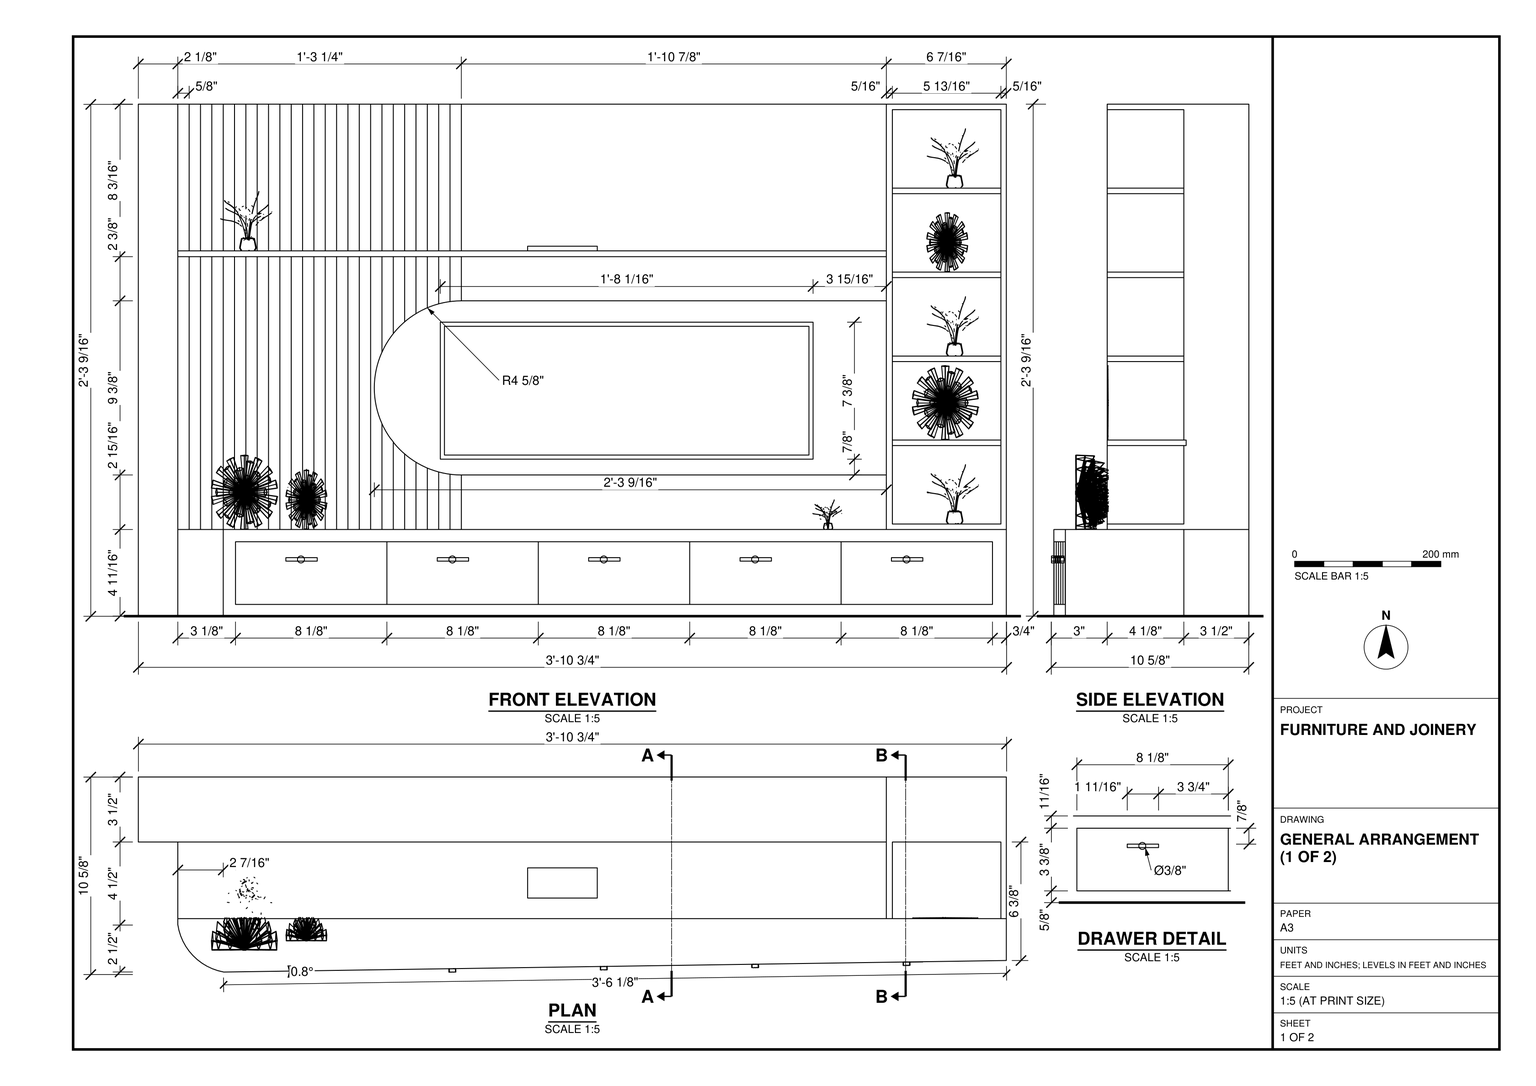
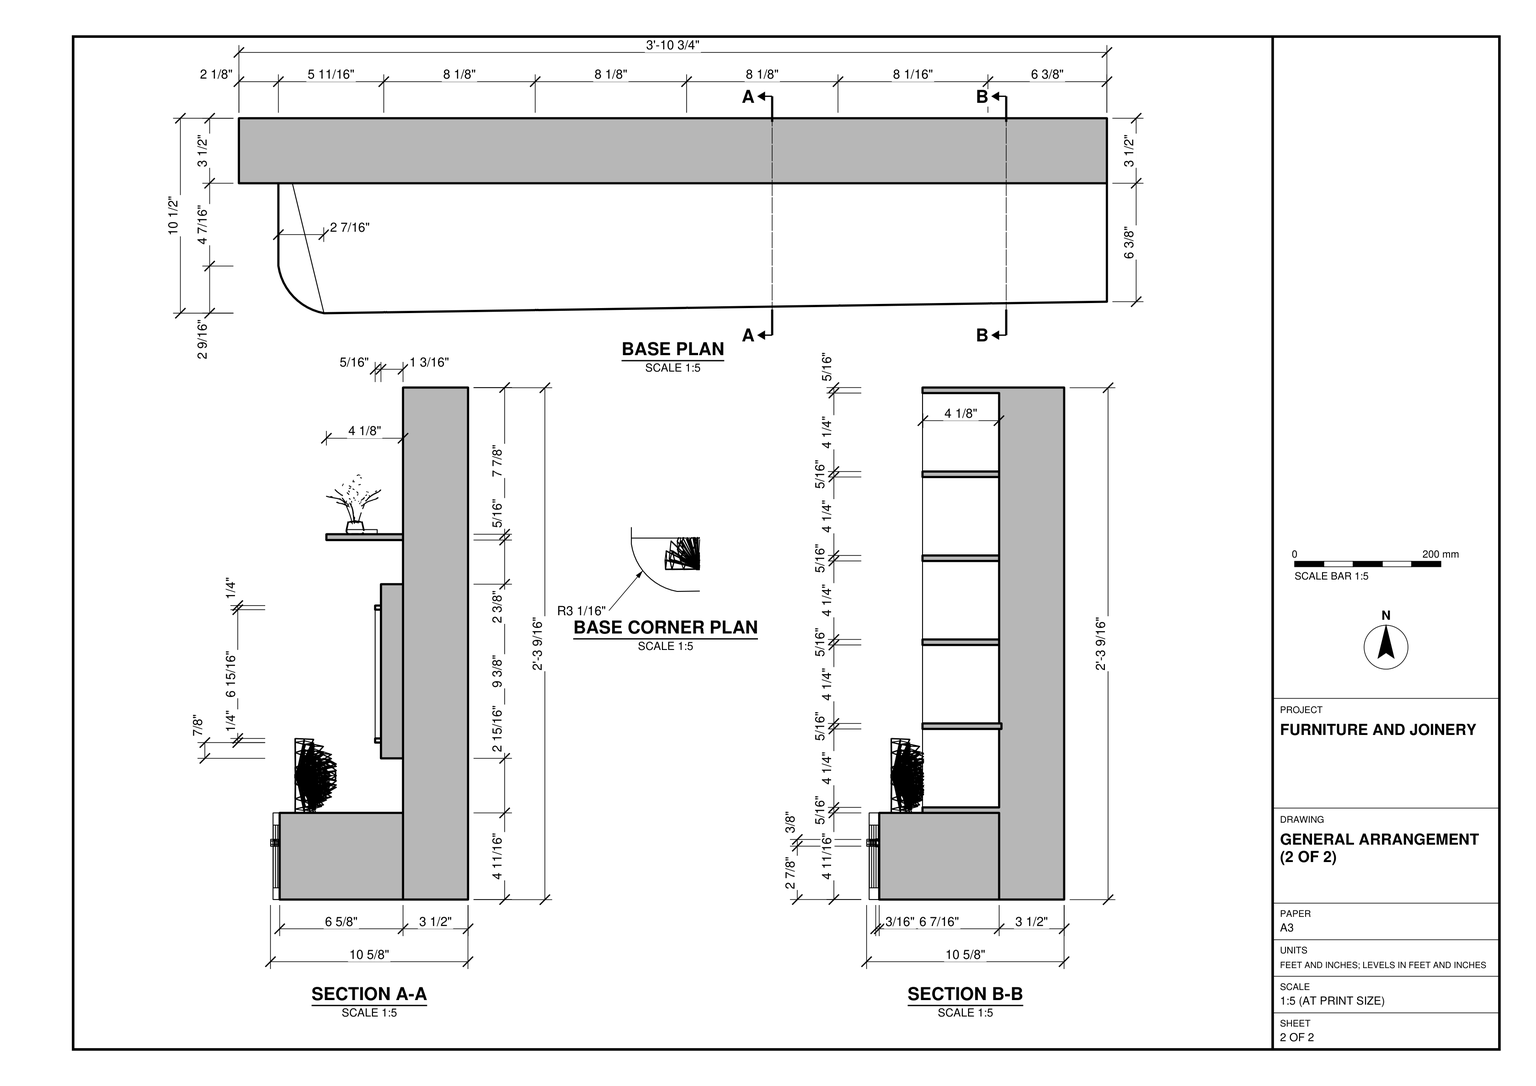
Build the media unit in SketchUp using task_files/diagram_01.pdf. Work in feet and inches. Set the underside of the base at ±0'-0" and make the complete unit 3'-10 3/4" wide, 10 5/8" deep and 2'-3 9/16" high. Use the front elevation for the face layout and the plans and sections for the profile and projection of each part.

Model the full-height backing and the low cabinet that projects in front of it. Follow the base plan at the rounded front-left corner and along the slightly angled front edge. Fit the five drawer fronts with horizontally centred pulls. Set out the vertical slats on the left, leaving the plain strip at the outer edge. Mount the framed rectangular screen on the projecting panel with the rounded left end. Run the thin shelf above the screen from the slatted area to the narrow shelving column on the right. Match the column's five open bays and shelf thicknesses to section B-B.

Plants and other loose display objects may be any suitable library components placed as shown. Keep distinct joinery pieces and the screen assembly in separate groups or components, and use components for repeated parts. Save one SketchUp model as output_files/media_unit_with_drawers_and_display_shelves.skp.

# SketchUp Ruby script. Lengths in inches.
U = 1.inch
M = Sketchup.active_model
def pt(a) = Geom::Point3d.new(a.map { |v| v * U })
def face(e, loops, mat)
  f = e.add_face(loops[0].map { |a| pt(a) })
  loops[1..].each { |l| e.add_face(l.map { |a| pt(a) }).erase! }
  f.material = f.back_material = mat if mat
  f
end
# faces: each face lists its corners as indices into pts; further lists are holes
def faces(e, pts, list, mat = nil) = list.each { |f| face(e, (f[0].is_a?(Array) ? f : [f]).map { |l| l.map { |i| pts[i] } }, mat) }
# xy, xz, yz: faces in a plane at the given z, y or x. An outline is a flat list of corners, or four numbers for a rectangle; further outlines are holes
def ring(l) = l.size == 4 ? [[l[0], l[1]], [l[2], l[1]], [l[2], l[3]], [l[0], l[3]]] : l.each_slice(2).to_a
def flat(e, list, mat, &to3) = list.each { |f| face(e, (f[0].is_a?(Array) ? f : [f]).map { |l| ring(l).map { |u, v| to3.(u, v) } }, mat) }
def xy(e, z, list, mat = nil) = flat(e, list, mat) { |x, y| [x, y, z] }
def xz(e, y, list, mat = nil) = flat(e, list, mat) { |x, z| [x, y, z] }
def yz(e, x, list, mat = nil) = flat(e, list, mat) { |y, z| [x, y, z] }
def lines(e, pts, list) = list.each { |a, b| e.add_line(pt(pts[a]), pt(pts[b])) }
# prism: a flat outline (further loops are holes) pulled along v
def prism(e, loops, v, mat = nil)
  f = face(e, loops, mat); d = Geom::Vector3d.new(v.map { |x| x * U })
  f.pushpull(f.normal.samedirection?(d) ? d.length : -d.length)
end
def box(e, o, s, mat = nil) = prism(e, [[o, [o[0] + s[0], o[1], o[2]], [o[0] + s[0], o[1] + s[1], o[2]], [o[0], o[1] + s[1], o[2]]]], [0, 0, s[2]], mat)
def at(x, y, z, deg = 0) = Geom::Transformation.translation(pt([x, y, z])) * Geom::Transformation.rotation(ORIGIN, Z_AXIS, deg.degrees)
def axes(o, x, y, z) = Geom::Transformation.new([*x, 0, *y, 0, *z, 0, *pt(o).to_a, 1])
def part(name) = M.definitions.add(name)
# library, detail: a bought-in or finely detailed component or shape, given as its bounding box
def library(name, o, s) = part(name).tap { |d| box(d.entities, o, s) }
def detail(e, o, s) = box(e.add_group.entities, o, s)
def put(e, d, t, mat = nil) = e.add_instance(d, t).tap { |i| i.material = mat if mat }
def group(e, t, mat = nil) = e.add_group.tap { |g| g.transformation = t; g.material = mat if mat }.entities
root = M.entities
M.materials.add("[0128_White]").color = [255, 255, 255]
M.materials.add("[0137_Black]").color = [0, 0, 0]
M.materials.add("[Carrera Marble]").color = [244, 244, 244]
M.materials.add("[Carrera Marble]1").color = [229, 229, 229]
M.materials.add("[Granite Dark Gray]").color = [69, 68, 68]
M.materials.add("[Wood Bamboo]").color = [165, 98, 40]
c1 = library("Group12\#2",[-37.1,-59.89,0],[61.11,59.71,94.13])
c2 = library("Groupe0\#1",[-19.63,20.99,0],[39.26,39.69,9.86])
xy(root,11.032,[[4.579,0.129,4.273,0.202,3.977,0.306,3.693,0.441,3.424,0.604,3.173,0.794,2.944,1.009,2.738,1.246,2.557,1.504,2.404,1.778,2.28,2.067,2.187,2.368,2.125,2.676,2.125,7.125,2.876,7.125],[4.579,0.129,2.876,7.125,46.722,7.125,46.722,0.75],[0,7.125,46.722,10.625]])
xy(root,15.696,[[4.579,0.129,46.722,0.75,46.722,3,40.263,3,40.263,7.125,2.125,7.125,2.125,2.676,2.187,2.368,2.28,2.067,2.404,1.778,2.557,1.504,2.738,1.246,2.944,1.009,3.173,0.794,3.424,0.604,3.693,0.441,3.977,0.306,4.273,0.202],[40.263,3,40.587,7.125],[40.587,3,46.43,7.125],[46.43,3,46.722,7.125]])
xy(root,15.991,[[40.587,3,46.43,7.125]],"[Wood Bamboo]")
xy(root,18.632,[[17.388,5.937,40.263,7.125]])
xy(root,19.483,[[16.256,5.625,36.319,5.937]],"[0137_Black]")
xy(root,19.704,[[16.477,5.625,36.098,5.937]],"[0137_Black]")
xy(root,20.216,[[40.587,7.125,46.43,7.25]])
xy(root,20.216,[[40.587,3,46.43,7.125]],"[Wood Bamboo]")
xy(root,20.512,[[40.587,7.125,46.43,7.25]])
xy(root,20.512,[[40.587,3,46.43,7.125]],"[Wood Bamboo]")
xy(root,24.737,[[40.587,3,46.43,7.125]],"[Wood Bamboo]")
xy(root,25.033,[[40.587,3,46.43,7.125]],"[Wood Bamboo]")
xy(root,26.637,[[16.477,5.625,36.098,5.937]],"[0137_Black]")
xy(root,26.858,[[16.256,5.625,36.319,5.937]],"[0137_Black]")
xy(root,28.007,[[17.388,5.937,40.263,7.125]])
xy(root,29.257,[[40.587,3,46.43,7.125]],"[Wood Bamboo]")
xy(root,29.553,[[40.587,3,46.43,7.125]],"[Wood Bamboo]")
xy(root,30.385,[[2.125,3,40.263,7.125]])
xy(root,30.698,[[[2.125,3,40.263,7.125],[20.954,4.108,24.704,5.733]],[20.954,4.108,24.704,5.733]])
xy(root,30.948,[[20.954,4.108,24.704,5.733]],"[Granite Dark Gray]")
xy(root,33.778,[[40.587,3,46.43,7.125]],"[Wood Bamboo]")
xy(root,34.074,[[40.587,3,46.43,7.125]],"[Wood Bamboo]")
xy(root,38.298,[[40.587,3,46.43,7.125]],"[Wood Bamboo]")
xy(root,38.594,[[0,7.125,40.263,10.625]])
xy(root,38.594,[[40.263,3,46.722,10.625]],"[Wood Bamboo]")
xz(root,3,[[2.125,30.385,40.263,30.698]])
xz(root,3,[[[40.263,15.696,46.722,38.594],[40.587,15.991,46.43,38.298]],[40.587,20.216,46.43,20.512],[40.587,24.737,46.43,25.033],[40.587,29.257,46.43,29.553],[40.587,33.778,46.43,34.074]],"[Wood Bamboo]")
xz(root,4.108,[[20.954,30.698,24.704,30.948]],"[Granite Dark Gray]")
xz(root,5.625,[[[16.256,19.483,36.319,26.858],[16.477,19.704,36.098,26.637]]],"[0137_Black]")
xz(root,5.733,[[20.954,30.698,24.704,30.948]])
xz(root,5.937,[[[16.256,19.483,36.319,26.858],[16.477,19.704,36.098,26.637]]])
xz(root,5.937,[[16.477,19.704,36.098,26.637]],"[0137_Black]")
xz(root,5.937,[[[17.388,18.632,40.263,18.632,40.263,28.007,17.388,28.007,17.142,28,16.898,27.981,16.777,27.965,16.654,27.949,16.413,27.904,16.174,27.847,16.167,27.845,15.939,27.777,15.708,27.695,15.556,27.633,15.481,27.602,15.259,27.496,15.044,27.379,14.946,27.319,14.835,27.251,14.632,27.112,14.4375,26.962,14.335,26.875,14.251,26.803,14.073,26.634,13.904,26.456,13.745,26.269,13.725,26.243,13.595,26.075,13.456,25.872,13.328,25.663,13.211,25.447,13.114,25.244,13.105,25.226,13.011,24.999,12.929,24.768,12.86,24.533,12.802,24.294,12.758,24.053,12.726,23.809,12.706,23.565,12.7,23.319,12.706,23.074,12.726,22.829,12.758,22.586,12.802,22.345,12.86,22.106,12.929,21.871,13.011,21.639,13.105,21.413,13.114,21.394,13.211,21.191,13.328,20.976,13.456,20.766,13.595,20.564,13.725,20.396,13.745,20.369,13.904,20.183,14.073,20.005,14.251,19.836,14.335,19.764,14.4375,19.676,14.632,19.527,14.835,19.388,14.946,19.32,15.044,19.26,15.259,19.143,15.481,19.037,15.556,19.006,15.708,18.943,15.939,18.861,16.167,18.794,16.174,18.792,16.413,18.734,16.654,18.69,16.777,18.673,16.898,18.657,17.142,18.638],[16.256,19.483,36.319,26.858]]],"[Carrera Marble]")
xz(root,7.125,[[2.125,11.032,46.722,15.696],[17.388,18.632,17.142,18.638,16.898,18.657,16.777,18.673,16.654,18.69,16.413,18.734,16.174,18.792,16.167,18.794,15.939,18.861,15.708,18.943,15.556,19.006,15.481,19.037,15.259,19.143,15.044,19.26,14.946,19.32,14.835,19.388,14.632,19.527,14.4375,19.676,14.335,19.764,14.251,19.836,14.073,20.005,13.904,20.183,13.745,20.369,13.725,20.396,13.595,20.564,13.456,20.766,13.328,20.976,13.211,21.191,13.114,21.394,13.105,21.413,13.011,21.639,12.929,21.871,12.86,22.106,12.802,22.345,12.758,22.586,12.726,22.829,12.706,23.074,12.7,23.319,12.706,23.565,12.726,23.809,12.758,24.053,12.802,24.294,12.86,24.533,12.929,24.768,13.011,24.999,13.105,25.226,13.114,25.244,13.211,25.447,13.328,25.663,13.456,25.872,13.595,26.075,13.725,26.243,13.745,26.269,13.904,26.456,14.073,26.634,14.251,26.803,14.335,26.875,14.4375,26.962,14.632,27.112,14.835,27.251,14.946,27.319,15.044,27.379,15.259,27.496,15.481,27.602,15.556,27.633,15.708,27.695,15.939,27.777,16.167,27.845,16.174,27.847,16.413,27.904,16.654,27.949,16.777,27.965,16.898,27.981,17.142,28,17.388,28.007,40.263,28.007,40.263,18.632],[40.587,24.737,46.43,25.033],[40.587,29.257,46.43,29.553],[2.125,30.385,40.263,30.698],
  [40.587,33.778,46.43,34.074]])
xz(root,7.125,[[17.388,15.696,40.263,18.632],[17.388,28.007,40.263,30.385],[17.388,30.698,40.263,38.594]],"[Carrera Marble]")
xz(root,7.125,[[0,11.032,2.125,38.594],[2.125,15.696,2.736,30.385],[2.736,15.696,3.346,30.385],[3.346,15.696,3.957,30.385],[3.957,15.696,4.567,30.385],
  [4.567,15.696,5.178,30.385],[5.178,15.696,5.788,30.385],[5.788,15.696,6.399,30.385],[6.399,15.696,7.009,30.385],[7.009,15.696,7.62,30.385],
  [7.62,15.696,8.23,30.385],[8.23,15.696,8.841,30.385],[8.841,15.696,9.451,30.385],[9.451,15.696,10.062,30.385],[10.062,15.696,10.672,30.385],
  [10.672,15.696,11.283,30.385],[11.283,15.696,11.893,30.385],[11.893,15.696,12.504,30.385],[12.504,15.696,13.114,15.696,13.114,21.394,13.105,21.413,13.011,21.639,12.929,21.871,12.86,22.106,12.802,22.345,12.758,22.586,12.726,22.829,12.706,23.074,12.7,23.319,12.706,23.565,12.726,23.809,12.758,24.053,12.802,24.294,12.86,24.533,12.929,24.768,13.011,24.999,13.105,25.226,13.114,25.244,13.114,30.385,12.504,30.385],[13.114,15.696,13.725,15.696,13.725,20.396,13.595,20.564,13.456,20.766,13.328,20.976,13.211,21.191,13.114,21.394],
  [13.725,15.696,14.335,15.696,14.335,19.764,14.251,19.836,14.073,20.005,13.904,20.183,13.745,20.369,13.725,20.396],[14.335,15.696,14.946,15.696,14.946,19.32,14.835,19.388,14.632,19.527,14.4375,19.676,14.335,19.764],[14.946,15.696,15.556,15.696,15.556,19.006,15.481,19.037,15.259,19.143,15.044,19.26,14.946,19.32],[15.556,15.696,16.167,15.696,16.167,18.794,15.939,18.861,15.708,18.943,15.556,19.006],[16.167,15.696,16.777,15.696,16.777,18.673,16.654,18.69,16.413,18.734,16.174,18.792,16.167,18.794],
  [16.777,15.696,17.388,15.696,17.388,18.632,17.142,18.638,16.898,18.657,16.777,18.673],[40.587,15.991,46.43,20.216],[40.587,20.512,46.43,24.737],[40.587,25.033,46.43,29.257],[13.114,25.244,13.211,25.447,13.328,25.663,13.456,25.872,13.595,26.075,13.725,26.243,13.725,30.385,13.114,30.385],
  [13.725,26.243,13.745,26.269,13.904,26.456,14.073,26.634,14.251,26.803,14.335,26.875,14.335,30.385,13.725,30.385],[14.335,26.875,14.4375,26.962,14.632,27.112,14.835,27.251,14.946,27.319,14.946,30.385,14.335,30.385],[14.946,27.319,15.044,27.379,15.259,27.496,15.481,27.602,15.556,27.633,15.556,30.385,14.946,30.385],[15.556,27.633,15.708,27.695,15.939,27.777,16.167,27.845,16.167,30.385,15.556,30.385],[16.167,27.845,16.174,27.847,16.413,27.904,16.654,27.949,16.777,27.965,16.777,30.385,16.167,30.385],
  [16.777,27.965,16.898,27.981,17.142,28,17.388,28.007,17.388,30.385,16.777,30.385],[40.587,29.553,46.43,33.778],[2.125,30.698,2.736,38.594],[2.736,30.698,3.346,38.594],[3.346,30.698,3.957,38.594],
  [3.957,30.698,4.567,38.594],[4.567,30.698,5.178,38.594],[5.178,30.698,5.788,38.594],[5.788,30.698,6.399,38.594],[6.399,30.698,7.009,38.594],
  [7.009,30.698,7.62,38.594],[7.62,30.698,8.23,38.594],[8.23,30.698,8.841,38.594],[8.841,30.698,9.451,38.594],[9.451,30.698,10.062,38.594],
  [10.062,30.698,10.672,38.594],[10.672,30.698,11.283,38.594],[11.283,30.698,11.893,38.594],[11.893,30.698,12.504,38.594],[12.504,30.698,13.114,38.594],
  [13.114,30.698,13.725,38.594],[13.725,30.698,14.335,38.594],[14.335,30.698,14.946,38.594],[14.946,30.698,15.556,38.594],[15.556,30.698,16.167,38.594],
  [16.167,30.698,16.777,38.594],[16.777,30.698,17.388,38.594],[40.587,34.074,46.43,38.298]],"[Wood Bamboo]")
xz(root,7.25,[[40.587,20.216,46.43,20.512]])
xz(root,10.625,[[0,11.032,46.722,38.594]])
yz(root,0,[[7.125,11.032,10.625,38.594]])
yz(root,2.125,[[2.676,11.032,7.125,15.696],[3,30.385,7.125,30.698]])
yz(root,16.256,[[5.625,19.483,5.937,26.858]],"[0137_Black]")
yz(root,16.477,[[5.625,19.704,5.937,26.637]],"[0137_Black]")
yz(root,20.954,[[4.108,30.698,5.733,30.948]],"[Granite Dark Gray]")
yz(root,24.704,[[4.108,30.698,5.733,30.948]],"[Granite Dark Gray]")
yz(root,36.098,[[5.625,19.704,5.937,26.637]],"[0137_Black]")
yz(root,36.319,[[5.625,19.483,5.937,26.858]],"[0137_Black]")
yz(root,40.263,[[5.937,18.632,7.125,28.007],[3,30.385,7.125,30.698]])
yz(root,40.263,[[3,15.696,3,30.385,7.125,30.385,7.125,28.007,5.937,28.007,5.937,18.632,7.125,18.632,7.125,15.696],[3,30.698,7.125,38.594]],"[Wood Bamboo]")
yz(root,40.587,[[3,20.216,7.25,20.512],[3,24.737,7.125,25.033],[3,29.257,7.125,29.553],[3,33.778,7.125,34.074]])
yz(root,40.587,[[3,15.991,7.125,20.216],[3,20.512,7.125,24.737],[3,25.033,7.125,29.257],[3,29.553,7.125,33.778],[3,34.074,7.125,38.298]],"[Wood Bamboo]")
yz(root,46.43,[[3,20.216,7.25,20.512],[3,24.737,7.125,25.033],[3,29.257,7.125,29.553],[3,33.778,7.125,34.074]])
yz(root,46.43,[[3,15.991,7.125,20.216],[3,20.512,7.125,24.737],[3,25.033,7.125,29.257],[3,29.553,7.125,33.778],[3,34.074,7.125,38.298]],"[Wood Bamboo]")
yz(root,46.722,[[0.75,11.032,7.125,15.696],[7.125,11.032,10.625,15.696],[3,15.696,10.625,38.594]])
p = [[4.579,0.129,11.032],[4.579,0.129,15.696],[4.273,0.202,15.696],[4.273,0.202,11.032],[46.722,0.75,11.032],[46.722,0.75,15.696],
  [5.231,0.138,11.662],[5.231,0.138,15.037],[13.38,0.258,15.037],[21.529,0.378,15.037],[29.678,0.499,15.037],[37.827,0.619,15.037],
  [45.977,0.739,15.037],[45.977,0.739,11.662],[37.827,0.619,11.662],[29.678,0.499,11.662],[21.529,0.378,11.662],[13.38,0.258,11.662],
  [3.977,0.306,15.696],[3.977,0.306,11.032],[3.693,0.441,15.696],[3.693,0.441,11.032],[3.424,0.604,15.696],[3.424,0.604,11.032],
  [3.173,0.794,15.696],[3.173,0.794,11.032],[2.944,1.009,15.696],[2.944,1.009,11.032],[2.738,1.246,15.696],[2.738,1.246,11.032],
  [2.557,1.504,15.696],[2.557,1.504,11.032],[2.404,1.778,15.696],[2.404,1.778,11.032],[2.28,2.067,15.696],[2.28,2.067,11.032],
  [2.187,2.368,15.696],[2.187,2.368,11.032],[2.125,2.676,15.696],[2.125,2.676,11.032],[7.942,0.178,14.181],[8.591,0.188,14.181],
  [8.619,0.188,14.217],[8.658,0.189,14.247],[8.703,0.19,14.265],[8.752,0.19,14.272],[8.8,0.191,14.265],[8.846,0.192,14.247],
  [8.884,0.192,14.217],[8.912,0.193,14.181],[9.629,0.203,14.181],[9.629,0.203,13.993],[8.915,0.193,13.993],[8.914,0.193,13.99],
  [8.884,0.192,13.952],[8.846,0.192,13.922],[8.8,0.191,13.903],[8.752,0.19,13.897],[8.703,0.19,13.903],[8.658,0.189,13.922],
  [8.619,0.188,13.952],[8.589,0.188,13.99],[8.588,0.188,13.993],[7.942,0.178,13.993],[17.778,0.323,14.181],[17.778,0.323,13.993],
  [17.064,0.3125,13.993],[17.063,0.3125,13.99],[17.033,0.312,13.952],[16.995,0.312,13.922],[16.949,0.311,13.903],[16.901,0.31,13.897],
  [16.852,0.31,13.903],[16.807,0.309,13.922],[16.768,0.308,13.952],[16.739,0.308,13.99],[16.737,0.308,13.993],[16.091,0.298,13.993],
  [16.091,0.298,14.181],[16.741,0.308,14.181],[17.061,0.3125,14.181],[25.21,0.433,14.181],[25.927,0.443,14.181],[25.927,0.443,13.993],
  [25.214,0.433,13.993],[25.212,0.433,13.99],[25.183,0.432,13.952],[25.144,0.432,13.922],[25.099,0.431,13.903],[25.05,0.43,13.897],
  [25.002,0.43,13.903],[24.956,0.429,13.922],[24.917,0.428,13.952],[24.888,0.428,13.99],[24.887,0.428,13.993],[24.24,0.418,13.993],
  [24.24,0.418,14.181],[24.89,0.428,14.181],[33.359,0.553,14.181],[34.076,0.563,14.181],[34.076,0.563,13.993],[33.363,0.553,13.993],
  [33.362,0.553,13.99],[33.332,0.552,13.952],[33.293,0.552,13.922],[33.248,0.551,13.903],[33.199,0.55,13.897],[33.151,0.55,13.903],
  [33.105,0.549,13.922],[33.067,0.548,13.952],[33.037,0.548,13.99],[33.036,0.548,13.993],[32.389,0.538,13.993],[32.389,0.538,14.181],
  [33.039,0.548,14.181],[41.509,0.673,14.181],[42.226,0.683,14.181],[42.226,0.683,13.993],[41.512,0.673,13.993],[41.511,0.673,13.99],
  [41.481,0.672,13.952],[41.442,0.672,13.922],[41.397,0.671,13.903],[41.348,0.67,13.897],[41.3,0.67,13.903],[41.255,0.669,13.922],
  [41.216,0.668,13.952],[41.186,0.668,13.99],[41.185,0.668,13.993],[40.538,0.658,13.993],[40.538,0.658,14.181],[41.188,0.668,14.181],
  [8.917,0.005,13.99],[8.918,0.005,13.993],[8.936,0.005,14.036],[8.942,0.006,14.084],[8.936,0.005,14.133],[8.917,0.005,14.178],
  [8.915,0.005,14.181],[8.887,0.005,14.217],[8.848,0.004,14.247],[8.803,0.003,14.265],[8.755,0.003,14.272],[8.706,0.002,14.265],
  [8.661,0.001,14.247],[8.622,0.001,14.217],[8.594,0,14.181],[8.592,0,14.178],[8.573,0,14.133],[8.567,0,14.084],
  [8.573,0,14.036],[8.591,0,13.993],[8.592,0,13.99],[8.622,0.001,13.952],[8.661,0.001,13.922],[8.706,0.002,13.903],
  [8.755,0.003,13.897],[8.803,0.003,13.903],[8.848,0.004,13.922],[8.887,0.005,13.952],[17.066,0.125,13.99],[17.067,0.125,13.993],
  [17.085,0.125,14.036],[17.091,0.126,14.084],[17.085,0.125,14.133],[17.066,0.125,14.178],[17.064,0.125,14.181],[17.036,0.125,14.217],
  [16.997,0.124,14.247],[16.952,0.124,14.265],[16.904,0.123,14.272],[16.855,0.122,14.265],[16.81,0.121,14.247],[16.771,0.121,14.217],
  [16.743,0.12,14.181],[16.741,0.12,14.178],[16.723,0.12,14.133],[16.716,0.12,14.084],[16.723,0.12,14.036],[16.74,0.12,13.993],
  [16.741,0.12,13.99],[16.771,0.121,13.952],[16.81,0.121,13.922],[16.855,0.122,13.903],[16.904,0.123,13.897],[16.952,0.124,13.903],
  [16.997,0.124,13.922],[17.036,0.125,13.952],[24.959,0.241,13.922],[24.92,0.241,13.952],[25.215,0.245,13.99],[25.216,0.245,13.993],
  [25.234,0.246,14.036],[25.24,0.246,14.084],[25.234,0.246,14.133],[25.215,0.245,14.178],[25.213,0.245,14.181],[25.185,0.245,14.217],
  [25.147,0.244,14.247],[25.101,0.244,14.265],[25.053,0.243,14.272],[25.004,0.242,14.265],[24.959,0.241,14.247],[24.92,0.241,14.217],
  [24.892,0.24,14.181],[24.89,0.24,14.178],[24.872,0.24,14.133],[24.865,0.24,14.084],[24.872,0.24,14.036],[24.889,0.24,13.993],
  [24.89,0.24,13.99],[25.004,0.242,13.903],[25.053,0.243,13.897],[25.101,0.244,13.903],[25.147,0.244,13.922],[25.185,0.245,13.952],
  [33.364,0.365,13.99],[33.365,0.365,13.993],[33.383,0.366,14.036],[33.389,0.366,14.084],[33.383,0.366,14.133],[33.364,0.365,14.178],
  [33.362,0.365,14.181],[33.334,0.365,14.217],[33.296,0.364,14.247],[33.25,0.364,14.265],[33.202,0.363,14.272],[33.153,0.362,14.265],
  [33.108,0.362,14.247],[33.069,0.361,14.217],[33.042,0.361,14.181],[33.04,0.36,14.178],[33.021,0.36,14.133],[33.014,0.36,14.084],
  [33.021,0.36,14.036],[33.038,0.36,13.993],[33.04,0.36,13.99],[33.069,0.361,13.952],[33.108,0.362,13.922],[33.153,0.362,13.903],
  [33.202,0.363,13.897],[33.25,0.364,13.903],[33.296,0.364,13.922],[33.334,0.365,13.952],[41.513,0.485,13.99],[41.514,0.485,13.993],
  [41.532,0.486,14.036],[41.539,0.486,14.084],[41.532,0.486,14.133],[41.513,0.485,14.178],[41.511,0.485,14.181],[41.484,0.485,14.217],
  [41.445,0.484,14.247],[41.4,0.484,14.265],[41.351,0.483,14.272],[41.303,0.482,14.265],[41.257,0.482,14.247],[41.218,0.481,14.217],
  [41.191,0.481,14.181],[41.189,0.481,14.178],[41.17,0.48,14.133],[41.164,0.48,14.084],[41.17,0.48,14.036],[41.1875,0.481,13.993],
  [41.189,0.481,13.99],[41.218,0.481,13.952],[41.257,0.482,13.922],[41.303,0.482,13.903],[41.351,0.483,13.897],[41.4,0.484,13.903],
  [41.445,0.484,13.922],[41.484,0.485,13.952],[8.564,0.1875,14.084],[8.571,0.1875,14.036],[8.933,0.193,14.036],[8.939,0.193,14.084],
  [16.713,0.308,14.084],[16.72,0.308,14.036],[17.082,0.313,14.036],[17.088,0.313,14.084],[8.571,0.1875,14.133],[8.589,0.188,14.178],
  [8.914,0.193,14.178],[8.933,0.193,14.133],[24.869,0.428,14.036],[24.863,0.428,14.084],[25.231,0.433,14.036],[25.238,0.433,14.084],
  [16.72,0.308,14.133],[16.739,0.308,14.178],[17.082,0.313,14.133],[17.063,0.3125,14.178],[24.869,0.428,14.133],[24.888,0.428,14.178],
  [25.231,0.433,14.133],[25.212,0.433,14.178],[33.018,0.548,14.036],[33.012,0.548,14.084],[33.38,0.553,14.036],[33.387,0.553,14.084],
  [33.018,0.548,14.133],[33.037,0.548,14.178],[33.38,0.553,14.133],[33.362,0.553,14.178],[41.167,0.668,14.036],[41.161,0.668,14.084],
  [41.529,0.673,14.036],[41.536,0.673,14.084],[41.167,0.668,14.133],[41.186,0.668,14.178],[41.529,0.673,14.133],[41.511,0.673,14.178],
  [16.768,0.308,14.217],[16.852,0.31,14.265],[16.807,0.309,14.247],[16.995,0.312,14.247],[16.949,0.311,14.265],[17.033,0.312,14.217],
  [24.917,0.428,14.217],[24.956,0.429,14.247],[25.002,0.43,14.265],[25.144,0.432,14.247],[25.099,0.431,14.265],[25.183,0.432,14.217],
  [33.067,0.548,14.217],[33.151,0.55,14.265],[33.105,0.549,14.247],[33.293,0.552,14.247],[33.248,0.551,14.265],[33.332,0.552,14.217],
  [41.255,0.669,14.247],[41.216,0.668,14.217],[41.3,0.67,14.265],[41.442,0.672,14.247],[41.397,0.671,14.265],[41.481,0.672,14.217],
  [16.901,0.31,14.272],[25.05,0.43,14.272],[33.199,0.55,14.272],[41.348,0.67,14.272],[16.898,7.125,18.657],[17.142,7.125,18.638],
  [17.142,5.937,18.638],[16.898,5.937,18.657],[17.388,7.125,18.632],[17.388,5.937,18.632],[16.174,7.125,18.792],[16.413,7.125,18.734],
  [16.413,5.937,18.734],[16.174,5.937,18.792],[16.654,7.125,18.69],[16.654,5.937,18.69],[16.777,7.125,18.673],[16.777,5.937,18.673],
  [15.939,7.125,18.861],[16.167,7.125,18.794],[16.167,5.937,18.794],[15.939,5.937,18.861],[15.481,7.125,19.037],[15.556,7.125,19.006],
  [15.708,7.125,18.943],[15.708,5.937,18.943],[15.556,5.937,19.006],[15.481,5.937,19.037],[15.259,7.125,19.143],[15.259,5.937,19.143],
  [15.044,7.125,19.26],[15.044,5.937,19.26],[14.835,7.125,19.388],[14.946,7.125,19.32],[14.946,5.937,19.32],[14.835,5.937,19.388],
  [14.632,7.125,19.527],[14.632,5.937,19.527],[14.4375,7.125,19.676],[14.4375,5.937,19.676],[14.251,7.125,19.836],[14.335,7.125,19.764],
  [14.335,5.937,19.764],[14.251,5.937,19.836],[14.073,7.125,20.005],[14.073,5.937,20.005],[13.904,7.125,20.183],[13.904,5.937,20.183],
  [13.745,7.125,20.369],[13.745,5.937,20.369],[13.595,7.125,20.564],[13.725,7.125,20.396],[13.725,5.937,20.396],[13.595,5.937,20.564],
  [13.456,7.125,20.766],[13.456,5.937,20.766],[13.328,7.125,20.976],[13.328,5.937,20.976],[13.211,7.125,21.191],[13.211,5.937,21.191],
  [13.105,7.125,21.413],[13.114,7.125,21.394],[13.114,5.937,21.394],[13.105,5.937,21.413],[13.011,7.125,21.639],[13.011,5.937,21.639],
  [12.929,7.125,21.871],[12.929,5.937,21.871],[12.86,7.125,22.106],[12.86,5.937,22.106],[12.802,7.125,22.345],[12.802,5.937,22.345],
  [12.758,7.125,22.586],[12.758,5.937,22.586],[12.726,7.125,22.829],[12.726,5.937,22.829],[12.706,7.125,23.074],[12.706,5.937,23.074],
  [12.7,7.125,23.319],[12.7,5.937,23.319],[12.706,7.125,23.565],[12.706,5.937,23.565],[12.726,7.125,23.809],[12.726,5.937,23.809],
  [12.758,7.125,24.053],[12.758,5.937,24.053],[12.802,7.125,24.294],[12.802,5.937,24.294],[12.86,7.125,24.533],[12.86,5.937,24.533],
  [12.929,7.125,24.768],[12.929,5.937,24.768],[13.011,7.125,24.999],[13.011,5.937,24.999],[13.105,7.125,25.226],[13.105,5.937,25.226],
  [13.211,7.125,25.447],[13.114,7.125,25.244],[13.114,5.937,25.244],[13.211,5.937,25.447],[13.328,7.125,25.663],[13.328,5.937,25.663],
  [13.456,7.125,25.872],[13.456,5.937,25.872],[13.595,7.125,26.075],[13.595,5.937,26.075],[13.745,7.125,26.269],[13.725,7.125,26.243],
  [13.725,5.937,26.243],[13.745,5.937,26.269],[13.904,7.125,26.456],[13.904,5.937,26.456],[14.073,7.125,26.634],[14.073,5.937,26.634],
  [14.251,7.125,26.803],[14.251,5.937,26.803],[14.4375,7.125,26.962],[14.335,7.125,26.875],[14.335,5.937,26.875],[14.4375,5.937,26.962],
  [14.632,7.125,27.112],[14.632,5.937,27.112],[14.835,7.125,27.251],[14.835,5.937,27.251],[15.044,7.125,27.379],[14.946,7.125,27.319],
  [14.946,5.937,27.319],[15.044,5.937,27.379],[15.259,7.125,27.496],[15.259,5.937,27.496],[15.481,7.125,27.602],[15.481,5.937,27.602],
  [15.708,7.125,27.695],[15.556,7.125,27.633],[15.556,5.937,27.633],[15.708,5.937,27.695],[15.939,7.125,27.777],[15.939,5.937,27.777],
  [16.174,7.125,27.847],[16.167,7.125,27.845],[16.167,5.937,27.845],[16.174,5.937,27.847],[16.413,7.125,27.904],[16.413,5.937,27.904],
  [16.654,7.125,27.949],[16.654,5.937,27.949],[16.898,7.125,27.981],[16.777,7.125,27.965],[16.777,5.937,27.965],[16.898,5.937,27.981],
  [17.142,7.125,28],[17.142,5.937,28],[17.388,7.125,28.007],[17.388,5.937,28.007]]
faces(root,p,[[0,1,2,3],[[4,5,1,0],[6,7,8,9,10,11,12,13,14,15,16,17]],[3,2,18,19],[19,18,20,21],[21,20,22,23],[23,22,24,25],[25,24,26,27],[27,26,28,29],
  [29,28,30,31],[30,32,33,31],[32,34,35,33],[34,36,37,35],[36,38,39,37],[[16,15,10,9],[81,82,83,84,85,86,87,88,89,90,91,92,93,94,95,96,97]],[[15,14,11,10],[98,99,100,101,102,103,104,105,106,107,108,109,110,111,112,113,114]],[[12,11,14,13],[115,116,117,118,119,120,121,122,123,124,125,126,127,128,129,130,131]],
  [340,341,342,343],[341,344,345,342],[346,347,348,349],[347,350,351,348],[350,352,340,343,353,351],[354,355,346,349,356,357],[358,359,360,361,362,363],[360,354,357,361],
  [364,358,363,365],[366,364,365,367],[368,369,366,367,370,371],[372,368,371,373],[374,372,373,375],[376,377,374,375,378,379],[380,376,379,381],[382,380,381,383],
  [384,382,383,385],[386,387,384,385,388,389],[390,386,389,391],[392,390,391,393],[394,392,393,395],[396,397,394,395,398,399],[400,396,399,401],[402,400,401,403],
  [404,402,403,405],[406,404,405,407],[408,406,407,409],[410,408,409,411],[412,410,411,413],[414,412,413,415],[416,414,415,417],[418,416,417,419],
  [420,418,419,421],[422,420,421,423],[424,422,423,425],[426,424,425,427],[428,426,427,429],[430,428,429,431],[432,433,430,431,434,435],[436,432,435,437],
  [438,436,437,439],[440,438,439,441],[442,443,440,441,444,445],[446,442,445,447],[448,446,447,449],[450,448,449,451],[452,453,450,451,454,455],[456,452,455,457],
  [458,456,457,459],[460,461,458,459,462,463],[464,460,463,465],[466,464,465,467],[468,469,466,467,470,471],[472,468,471,473],[474,475,472,473,476,477],[478,474,477,479],
  [480,478,479,481],[482,483,480,481,484,485],[486,482,485,487],[488,486,487,489]])
faces(root,p,[[[6,17,8,7],[40,41,42,43,44,45,46,47,48,49,50,51,52,53,54,55,56,57,58,59,60,61,62,63]],[[17,16,9,8],[64,65,66,67,68,69,70,71,72,73,74,75,76,77,78,79,80]],[60,59,154,153],[59,58,155,154],[58,57,156,155],[57,56,157,156],[56,55,158,157],[55,54,159,158],
  [74,73,182,181],[73,72,183,182],[71,70,185,184],[72,71,184,183],[70,69,186,185],[69,68,187,186],[62,52,53,54,55,56,57,58,59,60,61],[92,91,188,189],
  [91,90,211,188],[90,89,212,211],[89,88,213,212],[88,87,214,213],[87,86,215,214],[66,76,75,74,73,72,71,70,69,68,67],[84,94,93,92,91,90,89,88,87,86,85],[109,108,238,237],
  [108,107,239,238],[105,104,242,241],[107,106,240,239],[106,105,241,240],[104,103,243,242],[101,111,110,109,108,107,106,105,104,103,102],[126,125,266,265],[125,124,267,266],
  [124,123,268,267],[123,122,269,268],[121,120,271,270],[122,121,270,269],[118,128,127,126,125,124,123,122,121,120,119],[62,61,152,151],[61,60,153,152],[54,53,132,159],
  [53,52,133,132],[75,74,181,180],[76,75,180,179],[68,67,160,187],[67,66,161,160],[94,93,210,209],[93,92,189,210],[85,84,191,190],
  [86,85,190,215],[110,109,237,236],[111,110,236,235],[103,102,216,243],[102,101,217,216],[127,126,265,264],[128,127,264,263],[119,118,245,244],
  [120,119,244,271],[43,42,145,144],[42,41,146,145],[44,43,144,143],[48,47,140,139],[47,46,141,140],[49,48,139,138],[312,79,174,173],
  [313,314,172,171],[314,312,173,172],[315,316,169,168],[317,315,168,167],[80,317,167,166],[49,41,42,43,44,45,46,47,48],[318,97,204,203],[319,318,203,202],
  [320,319,202,201],[321,322,199,198],[323,321,198,197],[81,323,197,196],[324,114,230,229],[325,326,228,227],[326,324,229,228],[327,328,225,224],
  [98,329,223,222],[329,327,224,223],[330,331,257,256],[331,131,258,257],[332,330,256,255],[333,334,253,252],[335,333,252,251],[115,335,251,250],
  [45,44,143,142],[46,45,142,141],[316,336,170,169],[336,313,171,170],[337,320,201,200],[322,337,200,199],[338,325,227,226],[328,338,226,225],
  [334,339,254,253],[339,332,255,254]],"[0128_White]")
faces(root,p,[[132,133,134,135,136,137,138,139,140,141,142,143,144,145,146,147,148,149,150,151,152,153,154,155,156,157,158,159],[160,161,162,163,164,165,166,167,168,169,170,171,172,173,174,175,176,177,178,179,180,181,182,183,184,185,186,187],[190,191,192,193,194,195,196,197,198,199,200,201,202,203,204,205,206,207,208,209,210,189,188,211,212,213,214,215],[216,217,218,219,220,221,222,223,224,225,226,227,228,229,230,231,232,233,234,235,236,237,238,239,240,241,242,243],[244,245,246,247,248,249,250,251,252,253,254,255,256,257,258,259,260,261,262,263,264,265,266,267,268,269,270,271]],"[Granite Dark Gray]")
faces(root,p,[[272,273,150,149],[273,62,151,150],[52,274,134,133],[274,275,135,134],[276,277,178,177],[277,76,179,178],[66,278,162,161],[278,279,163,162],
  [63,62,273,272,280,281,41,40],[50,49,282,283,275,274,52,51],[284,94,209,208],[285,284,208,207],[286,287,193,192],[84,286,192,191],[77,76,277,276,288,289,79,78],[76,66,278,279,290,291,80,79,289,288,276,277],
  [64,80,291,290,279,278,66,65],[95,94,284,285,292,293,97,96],[81,97,293,292,285,284,94,84,286,287,294,295],[82,81,295,294,287,286,84,83],[296,111,235,234],[297,296,234,233],[101,298,218,217],[298,299,219,218],
  [112,111,296,297,300,301,114,113],[111,101,298,299,302,303,98,114,301,300,297,296],[304,128,263,262],[305,304,262,261],[306,307,247,246],[118,306,246,245],[99,98,303,302,299,298,101,100],[129,128,304,305,308,309,131,130],
  [115,131,309,308,305,304,128,118,306,307,310,311],[116,115,311,310,307,306,118,117],[281,280,148,147],[280,272,149,148],[275,283,136,135],[283,282,137,136],[289,288,176,175],[288,276,177,176],
  [290,291,165,164],[279,290,164,163],[293,292,206,205],[292,285,207,206],[294,295,195,194],[287,294,194,193],[301,300,232,231],[300,297,233,232],
  [302,303,221,220],[299,302,220,219],[308,305,261,260],[309,308,260,259],[307,310,248,247],[310,311,249,248],[41,281,147,146],[282,49,138,137],
  [79,289,175,174],[291,80,166,165],[97,293,205,204],[295,81,196,195],[114,301,231,230],[303,98,222,221],[131,309,259,258],[311,115,250,249]],"[Carrera Marble]1")
put(root,c1,axes([6.11,5.93,30.7],[0.0453,0,0],[0,0.049,0],[0,0,0.03397]))
put(root,c1,axes([44.14,5.93,34.07],[0.0453,0,0],[0,0.049,0],[0,0,0.03397]))
put(root,c1,axes([44.14,5.93,15.99],[0.0453,0,0],[0,0.049,0],[0,0,0.03397]))
put(root,c2,axes([43.4375,3,26.64],[0.09038,0,0],[0,0,-0.10097],[0,0.22789,0]))
put(root,c2,axes([43.54,5.08,34.45],[0.05603,0,0],[0,0,-0.08078],[0,0.13901,0]))
put(root,c1,axes([44.14,5.93,25.03],[0.0453,0,0],[0,0.049,0],[0,0,0.03397]))
put(root,c1,axes([37.24,5.28,15.7],[0.02537,0,0],[0,0.0245,0],[0,0,0.01698]))
put(root,c2,axes([5.71,1.29,21.82],[0.09038,0,0],[0,0,-0.10097],[0,0.22789,0]))
put(root,c2,axes([9.05,1.8,20.6],[0.05603,0,0],[0,0,-0.08078],[0,0.13901,0]))
